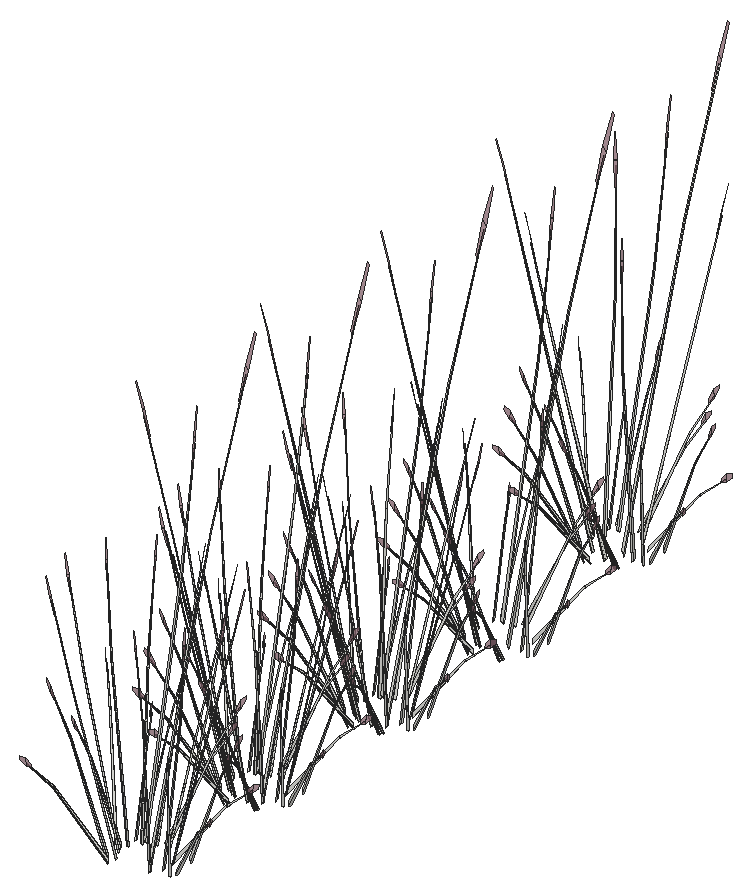
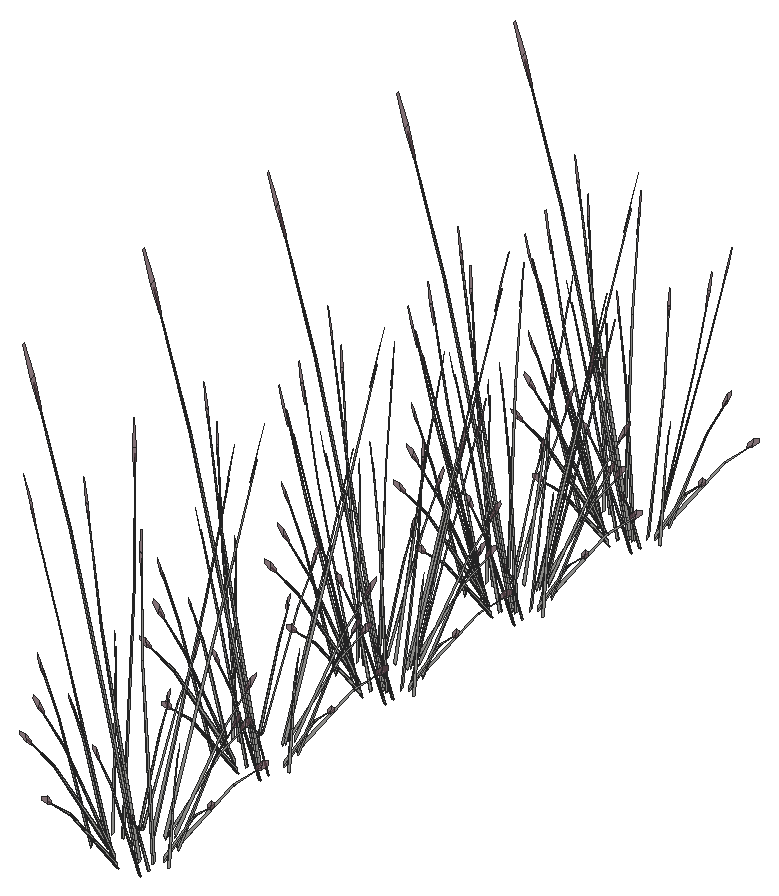
# SketchUp Ruby script. Lengths in inches.
U = 1.inch
M = Sketchup.active_model
def pt(a) = Geom::Point3d.new(a.map { |v| v * U })
def face(e, loops, mat)
  f = e.add_face(loops[0].map { |a| pt(a) })
  loops[1..].each { |l| e.add_face(l.map { |a| pt(a) }).erase! }
  f.material = f.back_material = mat if mat
  f
end
# faces: each face lists its corners as indices into pts; further lists are holes
def faces(e, pts, list, mat = nil) = list.each { |f| face(e, (f[0].is_a?(Array) ? f : [f]).map { |l| l.map { |i| pts[i] } }, mat) }
# xy, xz, yz: faces in a plane at the given z, y or x. An outline is a flat list of corners, or four numbers for a rectangle; further outlines are holes
def ring(l) = l.size == 4 ? [[l[0], l[1]], [l[2], l[1]], [l[2], l[3]], [l[0], l[3]]] : l.each_slice(2).to_a
def flat(e, list, mat, &to3) = list.each { |f| face(e, (f[0].is_a?(Array) ? f : [f]).map { |l| ring(l).map { |u, v| to3.(u, v) } }, mat) }
def xy(e, z, list, mat = nil) = flat(e, list, mat) { |x, y| [x, y, z] }
def xz(e, y, list, mat = nil) = flat(e, list, mat) { |x, z| [x, y, z] }
def yz(e, x, list, mat = nil) = flat(e, list, mat) { |y, z| [x, y, z] }
def lines(e, pts, list) = list.each { |a, b| e.add_line(pt(pts[a]), pt(pts[b])) }
# prism: a flat outline (further loops are holes) pulled along v
def prism(e, loops, v, mat = nil)
  f = face(e, loops, mat); d = Geom::Vector3d.new(v.map { |x| x * U })
  f.pushpull(f.normal.samedirection?(d) ? d.length : -d.length)
end
def box(e, o, s, mat = nil) = prism(e, [[o, [o[0] + s[0], o[1], o[2]], [o[0] + s[0], o[1] + s[1], o[2]], [o[0], o[1] + s[1], o[2]]]], [0, 0, s[2]], mat)
def at(x, y, z, deg = 0) = Geom::Transformation.translation(pt([x, y, z])) * Geom::Transformation.rotation(ORIGIN, Z_AXIS, deg.degrees)
def axes(o, x, y, z) = Geom::Transformation.new([*x, 0, *y, 0, *z, 0, *pt(o).to_a, 1])
def part(name) = M.definitions.add(name)
# library, detail: a bought-in or finely detailed component or shape, given as its bounding box
def library(name, o, s) = part(name).tap { |d| box(d.entities, o, s) }
def detail(e, o, s) = box(e.add_group.entities, o, s)
def put(e, d, t, mat = nil) = e.add_instance(d, t).tap { |i| i.material = mat if mat }
def group(e, t, mat = nil) = e.add_group.tap { |g| g.transformation = t; g.material = mat if mat }.entities
root = M.entities
M.materials.add("LightPink_Translucent").color = [144, 107, 117]
M.materials["LightPink_Translucent"].alpha = 0.75
c1 = part("blade")
p = [[2.15,0.21,22],[0,0.17,0],[0.09,0.45,0],[2.18,0.31,22],[2.29,0.31,22],[0.38,0.45,0],
  [2.48,0.24,33],[2.49,0.24,33],[2.48,0.22,33]]
faces(c1.entities,p,[[0,1,2,3],[4,5,2,3],[6,3,4,7],[8,0,3,6]])
c2 = part("seeds")
p = [[0.3,-0.1,1.38],[-0.01,-0.03,1.59],[-0.01,-0.03,0.03],[0.14,-0.07,-0.07],[0.29,-0.03,3],[0.15,0.01,3.11]]
faces(c2.entities,p,[[0,1,2,3],[1,0,4,5]],"LightPink_Translucent")
c3 = part("blade with seeds")
put(c3.entities,c1,at(0,0,0))
put(c3.entities,c2,axes([2.4,0.25,30.99],[1.5799,-0.05474,1.17369],[-0.12525,1.92788,0.29478],[-0.07173,-0.02425,1.56792]))
put(root,c3,axes([337.34,75.88,268.4],[0.42027,0.02533,0.05988],[-0.01152,0.38243,0.47138],[0.04398,-0.14649,0.71878]))
put(root,c3,axes([333.7,75.16,268.39],[-0.11004,-0.00384,1.62908],[-0.35032,0.38367,-0.25764],[-0.18692,-0.07839,0.13065]))
put(root,c3,axes([339.02,76.93,268.38],[-0.0668,-0.00413,1.65179],[-0.27738,-0.44233,-0.15608],[0.11139,-0.14544,0.29231]))
put(root,c3,axes([333.81,76.02,268.4],[0.02575,-0.41332,0.05988],[0.38885,0.01133,0.47138],[-0.14895,-0.04325,0.71878]))
put(root,c3,axes([338.03,76.95,268.4],[0.35109,0.22859,0.05988],[-0.2044,0.32553,0.47138],[0.11256,-0.10524,0.71878]))
put(root,c3,axes([339.28,77.46,268.39],[0.07097,-0.08279,1.62908],[-0.09083,-0.50786,-0.25764],[0.17806,-0.09629,0.13065]))
put(root,c3,axes([333.28,75.48,268.38],[0.03791,0.05424,1.65179],[-0.18278,0.48761,-0.15608],[-0.18511,0.00353,0.29231]))
put(root,c3,axes([333.21,77.15,268.4],[-0.18783,-0.37061,0.05988],[0.34252,-0.1814,0.47138],[-0.15099,0.03579,0.71878]))
put(root,c3,axes([338.09,78.22,268.4],[0.18783,0.37061,0.05988],[-0.34252,0.1814,0.47138],[0.15099,-0.03579,0.71878]))
put(root,c3,axes([338.9,79.7,268.38],[-0.04624,-0.04758,1.65179],[0.10116,-0.51007,-0.15608],[0.18215,-0.03259,0.29231]))
put(root,c3,axes([332.88,77.625,268.39],[-0.08351,0.07057,1.62908],[0.0071,0.51561,-0.25764],[-0.19143,0.06705,0.13065]))
put(root,c3,axes([337.75,78.92,268.39],[0.10971,-0.00919,1.62908],[0.30091,-0.42228,-0.25764],[0.19514,0.05574,0.13065]))
put(root,c3,axes([333.27,78.42,268.4],[-0.35109,-0.22859,0.05988],[0.2044,-0.32553,0.47138],[-0.11256,0.10524,0.71878]))
put(root,c3,axes([331.96,78.15,268.38],[0.06527,0.01458,1.65179],[0.20191,0.48025,-0.15608],[-0.1336,0.12605,0.29231]))
put(root,c3,axes([337.49,79.35,268.4],[-0.02575,0.41332,0.05988],[-0.38885,-0.01133,0.47138],[0.14895,0.04325,0.71878]))
put(root,c3,axes([336.625,77.11,268.17],[-0.44191,-0.28242,1.28769],[0.46662,-0.43971,0.5556],[0.14258,0.26499,1.24467]))
put(root,c3,axes([335.88,80.24,268.38],[0.00151,-0.06581,1.65179],[0.43826,-0.29033,-0.15608],[0.15223,0.10363,0.29231]))
put(root,c3,axes([333.96,79.49,268.4],[-0.42027,-0.02533,0.05988],[0.01152,-0.38243,0.47138],[-0.04398,0.14649,0.71878]))
put(root,c3,axes([336.39,80.03,268.4],[-0.23243,0.34529,0.05988],[-0.331,-0.20103,0.47138],[0.10701,0.1107,0.71878]))
put(root,c3,axes([335.1,80.08,268.4],[-0.37684,0.18473,0.05988],[-0.18445,-0.33686,0.47138],[0.03639,0.14849,0.71878]))
put(root,c3,axes([332.9,79.55,268.39],[-0.01271,0.10756,1.62908],[0.36076,0.37419,-0.25764],[-0.09444,0.17695,0.13065]))
put(root,c3,axes([334.05,79.31,269.03],[0.56206,0.02693,-0.12569],[-0.01536,0.50991,-0.69765],[-0.03904,0.19638,1.06006]))
put(root,c3,axes([332.86,80.65,268.38],[0.05802,-0.03282,1.65179],[0.47954,0.21828,-0.15608],[-0.01127,0.18175,0.29231]))
put(root,c3,axes([334.97,80.88,268.39],[0.06483,0.08753,1.62908],[0.52315,0.03439,-0.25764],[0.05261,0.19303,0.13065]))
put(root,c3,axes([335.41,89.2,268.39],[-0.07822,-0.07621,1.62908],[-0.52201,0.04832,-0.25764],[-0.08331,-0.18228,0.13065]))
put(root,c3,axes([337.76,90.14,268.39],[-0.00494,-0.10818,1.62908],[-0.41695,-0.31265,-0.25764],[0.06446,-0.18952,0.13065]))
put(root,c3,axes([337.65,89.75,268.38],[-0.05194,0.04152,1.65179],[-0.50886,-0.14007,-0.15608],[-0.01842,-0.18118,0.29231]))
put(root,c3,axes([334.88,88.95,268.38],[-0.00954,0.06515,1.65179],[-0.47055,0.23645,-0.15608],[-0.13847,-0.12087,0.29231]))
put(root,c3,axes([336.2,90.18,268.4],[0.37684,-0.18473,0.05988],[0.18445,0.33686,0.47138],[-0.03639,-0.14849,0.71878]))
put(root,c3,axes([334.91,90.23,268.4],[0.23243,-0.34529,0.05988],[0.331,0.20103,0.47138],[-0.10701,-0.1107,0.71878]))
put(root,c3,axes([335.01,90.19,269.06],[-0.34131,0.52108,-0.12682],[-0.49429,-0.3002,-0.70393],[-0.17182,-0.14722,1.06961]))
put(root,c3,axes([337.34,90.77,268.4],[0.42027,0.02533,0.05988],[-0.01152,0.38243,0.47138],[0.04398,-0.14649,0.71878]))
put(root,c3,axes([333.7,90.04,268.39],[-0.11004,-0.00384,1.62908],[-0.35032,0.38367,-0.25764],[-0.18692,-0.07839,0.13065]))
put(root,c3,axes([339.02,91.82,268.38],[-0.0668,-0.00413,1.65179],[-0.27738,-0.44233,-0.15608],[0.11139,-0.14544,0.29231]))
put(root,c3,axes([333.81,90.91,268.4],[0.02575,-0.41332,0.05988],[0.38885,0.01133,0.47138],[-0.14895,-0.04325,0.71878]))
put(root,c3,axes([338.03,91.84,268.4],[0.35109,0.22859,0.05988],[-0.2044,0.32553,0.47138],[0.11256,-0.10524,0.71878]))
put(root,c3,axes([339.28,92.35,268.39],[0.07097,-0.08279,1.62908],[-0.09083,-0.50786,-0.25764],[0.17806,-0.09629,0.13065]))
put(root,c3,axes([333.28,90.37,268.38],[0.03791,0.05424,1.65179],[-0.18278,0.48761,-0.15608],[-0.18511,0.00353,0.29231]))
put(root,c3,axes([333.21,92.03,268.4],[-0.18783,-0.37061,0.05988],[0.34252,-0.1814,0.47138],[-0.15099,0.03579,0.71878]))
put(root,c3,axes([338.09,93.11,268.4],[0.18783,0.37061,0.05988],[-0.34252,0.1814,0.47138],[0.15099,-0.03579,0.71878]))
put(root,c3,axes([338.9,94.58,268.38],[-0.04624,-0.04758,1.65179],[0.10116,-0.51007,-0.15608],[0.18215,-0.03259,0.29231]))
put(root,c3,axes([332.88,92.51,268.39],[-0.08351,0.07057,1.62908],[0.0071,0.51561,-0.25764],[-0.19143,0.06705,0.13065]))
put(root,c3,axes([337.75,93.8125,268.39],[0.10971,-0.00919,1.62908],[0.30091,-0.42228,-0.25764],[0.19514,0.05574,0.13065]))
put(root,c3,axes([333.27,93.3,268.4],[-0.35109,-0.22859,0.05988],[0.2044,-0.32553,0.47138],[-0.11256,0.10524,0.71878]))
put(root,c3,axes([331.96,93.03,268.38],[0.06527,0.01458,1.65179],[0.20191,0.48025,-0.15608],[-0.1336,0.12605,0.29231]))
put(root,c3,axes([337.49,94.24,268.4],[-0.02575,0.41332,0.05988],[-0.38885,-0.01133,0.47138],[0.14895,0.04325,0.71878]))
put(root,c3,axes([336.625,92,268.17],[-0.44191,-0.28242,1.28769],[0.46662,-0.43971,0.5556],[0.14258,0.26499,1.24467]))
put(root,c3,axes([335.88,95.13,268.38],[0.00151,-0.06581,1.65179],[0.43826,-0.29033,-0.15608],[0.15223,0.10363,0.29231]))
put(root,c3,axes([333.96,94.375,268.4],[-0.42027,-0.02533,0.05988],[0.01152,-0.38243,0.47138],[-0.04398,0.14649,0.71878]))
put(root,c3,axes([336.39,94.91,268.4],[-0.23243,0.34529,0.05988],[-0.331,-0.20103,0.47138],[0.10701,0.1107,0.71878]))
put(root,c3,axes([335.1,94.97,268.4],[-0.37684,0.18473,0.05988],[-0.18445,-0.33686,0.47138],[0.03639,0.14849,0.71878]))
put(root,c3,axes([332.9,94.4375,268.39],[-0.01271,0.10756,1.62908],[0.36076,0.37419,-0.25764],[-0.09444,0.17695,0.13065]))
put(root,c3,axes([334.05,94.2,269.03],[0.56206,0.02693,-0.12569],[-0.01536,0.50991,-0.69765],[-0.03904,0.19638,1.06006]))
put(root,c3,axes([332.86,95.54,268.38],[0.05802,-0.03282,1.65179],[0.47954,0.21828,-0.15608],[-0.01127,0.18175,0.29231]))
put(root,c3,axes([334.97,95.77,268.39],[0.06483,0.08753,1.62908],[0.52315,0.03439,-0.25764],[0.05261,0.19303,0.13065]))
put(root,c3,axes([335.41,105.62,268.39],[-0.07822,-0.07621,1.62908],[-0.52201,0.04832,-0.25764],[-0.08331,-0.18228,0.13065]))
put(root,c3,axes([337.76,106.56,268.39],[-0.00494,-0.10818,1.62908],[-0.41695,-0.31265,-0.25764],[0.06446,-0.18952,0.13065]))
put(root,c3,axes([337.65,106.17,268.38],[-0.05194,0.04152,1.65179],[-0.50886,-0.14007,-0.15608],[-0.01842,-0.18118,0.29231]))
put(root,c3,axes([334.88,105.37,268.38],[-0.00954,0.06515,1.65179],[-0.47055,0.23645,-0.15608],[-0.13847,-0.12087,0.29231]))
put(root,c3,axes([336.2,106.59,268.4],[0.37684,-0.18473,0.05988],[0.18445,0.33686,0.47138],[-0.03639,-0.14849,0.71878]))
put(root,c3,axes([334.91,106.65,268.4],[0.23243,-0.34529,0.05988],[0.331,0.20103,0.47138],[-0.10701,-0.1107,0.71878]))
put(root,c3,axes([335.01,106.61,269.06],[-0.34131,0.52108,-0.12682],[-0.49429,-0.3002,-0.70393],[-0.17182,-0.14722,1.06961]))
put(root,c3,axes([337.34,107.18,268.4],[0.42027,0.02533,0.05988],[-0.01152,0.38243,0.47138],[0.04398,-0.14649,0.71878]))
put(root,c3,axes([333.7,106.46,268.39],[-0.11004,-0.00384,1.62908],[-0.35032,0.38367,-0.25764],[-0.18692,-0.07839,0.13065]))
put(root,c3,axes([339.02,108.24,268.38],[-0.0668,-0.00413,1.65179],[-0.27738,-0.44233,-0.15608],[0.11139,-0.14544,0.29231]))
put(root,c3,axes([333.81,107.33,268.4],[0.02575,-0.41332,0.05988],[0.38885,0.01133,0.47138],[-0.14895,-0.04325,0.71878]))
put(root,c3,axes([338.03,108.26,268.4],[0.35109,0.22859,0.05988],[-0.2044,0.32553,0.47138],[0.11256,-0.10524,0.71878]))
put(root,c3,axes([339.28,108.77,268.39],[0.07097,-0.08279,1.62908],[-0.09083,-0.50786,-0.25764],[0.17806,-0.09629,0.13065]))
put(root,c3,axes([333.28,106.79,268.38],[0.03791,0.05424,1.65179],[-0.18278,0.48761,-0.15608],[-0.18511,0.00353,0.29231]))
put(root,c3,axes([333.21,108.45,268.4],[-0.18783,-0.37061,0.05988],[0.34252,-0.1814,0.47138],[-0.15099,0.03579,0.71878]))
put(root,c3,axes([338.09,109.53,268.4],[0.18783,0.37061,0.05988],[-0.34252,0.1814,0.47138],[0.15099,-0.03579,0.71878]))
put(root,c3,axes([338.9,111,268.38],[-0.04624,-0.04758,1.65179],[0.10116,-0.51007,-0.15608],[0.18215,-0.03259,0.29231]))
put(root,c3,axes([332.88,108.93,268.39],[-0.08351,0.07057,1.62908],[0.0071,0.51561,-0.25764],[-0.19143,0.06705,0.13065]))
put(root,c3,axes([337.75,110.23,268.39],[0.10971,-0.00919,1.62908],[0.30091,-0.42228,-0.25764],[0.19514,0.05574,0.13065]))
put(root,c3,axes([333.27,109.72,268.4],[-0.35109,-0.22859,0.05988],[0.2044,-0.32553,0.47138],[-0.11256,0.10524,0.71878]))
put(root,c3,axes([331.96,109.45,268.38],[0.06527,0.01458,1.65179],[0.20191,0.48025,-0.15608],[-0.1336,0.12605,0.29231]))
put(root,c3,axes([337.49,110.65,268.4],[-0.02575,0.41332,0.05988],[-0.38885,-0.01133,0.47138],[0.14895,0.04325,0.71878]))
put(root,c3,axes([336.625,108.42,268.17],[-0.44191,-0.28242,1.28769],[0.46662,-0.43971,0.5556],[0.14258,0.26499,1.24467]))
put(root,c3,axes([335.88,111.55,268.38],[0.00151,-0.06581,1.65179],[0.43826,-0.29033,-0.15608],[0.15223,0.10363,0.29231]))
put(root,c3,axes([333.96,110.79,268.4],[-0.42027,-0.02533,0.05988],[0.01152,-0.38243,0.47138],[-0.04398,0.14649,0.71878]))
put(root,c3,axes([336.39,111.33,268.4],[-0.23243,0.34529,0.05988],[-0.331,-0.20103,0.47138],[0.10701,0.1107,0.71878]))
put(root,c3,axes([335.1,111.38,268.4],[-0.37684,0.18473,0.05988],[-0.18445,-0.33686,0.47138],[0.03639,0.14849,0.71878]))
put(root,c3,axes([332.9,110.86,268.39],[-0.01271,0.10756,1.62908],[0.36076,0.37419,-0.25764],[-0.09444,0.17695,0.13065]))
put(root,c3,axes([334.05,110.61,269.03],[0.56206,0.02693,-0.12569],[-0.01536,0.50991,-0.69765],[-0.03904,0.19638,1.06006]))
put(root,c3,axes([332.86,111.96,268.38],[0.05802,-0.03282,1.65179],[0.47954,0.21828,-0.15608],[-0.01127,0.18175,0.29231]))
put(root,c3,axes([334.97,112.1875,268.39],[0.06483,0.08753,1.62908],[0.52315,0.03439,-0.25764],[0.05261,0.19303,0.13065]))
put(root,c3,axes([335.41,121.46,268.39],[-0.07822,-0.07621,1.62908],[-0.52201,0.04832,-0.25764],[-0.08331,-0.18228,0.13065]))
put(root,c3,axes([337.76,122.39,268.39],[-0.00494,-0.10818,1.62908],[-0.41695,-0.31265,-0.25764],[0.06446,-0.18952,0.13065]))
put(root,c3,axes([337.65,122.01,268.38],[-0.05194,0.04152,1.65179],[-0.50886,-0.14007,-0.15608],[-0.01842,-0.18118,0.29231]))
put(root,c3,axes([334.88,121.21,268.38],[-0.00954,0.06515,1.65179],[-0.47055,0.23645,-0.15608],[-0.13847,-0.12087,0.29231]))
put(root,c3,axes([334.91,122.49,268.4],[0.23243,-0.34529,0.05988],[0.331,0.20103,0.47138],[-0.10701,-0.1107,0.71878]))
put(root,c3,axes([335.01,122.45,269.06],[-0.34131,0.52108,-0.12682],[-0.49429,-0.3002,-0.70393],[-0.17182,-0.14722,1.06961]))
put(root,c3,axes([333.7,122.3,268.39],[-0.11004,-0.00384,1.62908],[-0.35032,0.38367,-0.25764],[-0.18692,-0.07839,0.13065]))
put(root,c3,axes([339.02,124.08,268.38],[-0.0668,-0.00413,1.65179],[-0.27738,-0.44233,-0.15608],[0.11139,-0.14544,0.29231]))
put(root,c3,axes([338.03,124.1,268.4],[0.35109,0.22859,0.05988],[-0.2044,0.32553,0.47138],[0.11256,-0.10524,0.71878]))
put(root,c3,axes([339.28,124.61,268.39],[0.07097,-0.08279,1.62908],[-0.09083,-0.50786,-0.25764],[0.17806,-0.09629,0.13065]))
put(root,c3,axes([333.28,122.625,268.38],[0.03791,0.05424,1.65179],[-0.18278,0.48761,-0.15608],[-0.18511,0.00353,0.29231]))
put(root,c3,axes([338.9,126.84,268.38],[-0.04624,-0.04758,1.65179],[0.10116,-0.51007,-0.15608],[0.18215,-0.03259,0.29231]))
put(root,c3,axes([332.88,124.77,268.39],[-0.08351,0.07057,1.62908],[0.0071,0.51561,-0.25764],[-0.19143,0.06705,0.13065]))
put(root,c3,axes([337.75,126.07,268.39],[0.10971,-0.00919,1.62908],[0.30091,-0.42228,-0.25764],[0.19514,0.05574,0.13065]))
put(root,c3,axes([331.96,125.29,268.38],[0.06527,0.01458,1.65179],[0.20191,0.48025,-0.15608],[-0.1336,0.12605,0.29231]))
put(root,c3,axes([336.625,124.26,268.17],[-0.44191,-0.28242,1.28769],[0.46662,-0.43971,0.5556],[0.14258,0.26499,1.24467]))
put(root,c3,axes([335.88,127.39,268.38],[0.00151,-0.06581,1.65179],[0.43826,-0.29033,-0.15608],[0.15223,0.10363,0.29231]))
put(root,c3,axes([335.1,127.22,268.4],[-0.37684,0.18473,0.05988],[-0.18445,-0.33686,0.47138],[0.03639,0.14849,0.71878]))
put(root,c3,axes([332.9,126.7,268.39],[-0.01271,0.10756,1.62908],[0.36076,0.37419,-0.25764],[-0.09444,0.17695,0.13065]))
put(root,c3,axes([334.05,126.45,269.03],[0.56206,0.02693,-0.12569],[-0.01536,0.50991,-0.69765],[-0.03904,0.19638,1.06006]))
put(root,c3,axes([332.86,127.8,268.38],[0.05802,-0.03282,1.65179],[0.47954,0.21828,-0.15608],[-0.01127,0.18175,0.29231]))
put(root,c3,axes([334.97,128.03,268.39],[0.06483,0.08753,1.62908],[0.52315,0.03439,-0.25764],[0.05261,0.19303,0.13065]))
put(root,c3,axes([333.2,139.47,268.39],[-0.07822,-0.07621,1.62908],[-0.52201,0.04832,-0.25764],[-0.08331,-0.18228,0.13065]))
put(root,c3,axes([335.54,140.4,268.39],[-0.00494,-0.10818,1.62908],[-0.41695,-0.31265,-0.25764],[0.06446,-0.18952,0.13065]))
put(root,c3,axes([335.43,140.02,268.38],[-0.05194,0.04152,1.65179],[-0.50886,-0.14007,-0.15608],[-0.01842,-0.18118,0.29231]))
put(root,c3,axes([332.66,139.22,268.38],[-0.00954,0.06515,1.65179],[-0.47055,0.23645,-0.15608],[-0.13847,-0.12087,0.29231]))
put(root,c3,axes([333.99,140.65,268.6875],[-0.50045,0.25306,-0.11324],[-0.24593,-0.44915,-0.62851],[-0.06603,-0.18927,0.95501]))
put(root,c3,axes([332.8,140.46,269.06],[-0.34131,0.52108,-0.12682],[-0.49429,-0.3002,-0.70393],[-0.17182,-0.14722,1.06961]))
put(root,c3,axes([331.49,140.31,268.39],[-0.11004,-0.00384,1.62908],[-0.35032,0.38367,-0.25764],[-0.18692,-0.07839,0.13065]))
put(root,c3,axes([335.64,142.22,268.6875],[-0.47307,-0.29971,-0.11324],[0.27254,-0.43404,-0.62851],[0.13365,-0.15087,0.95501]))
put(root,c3,axes([336.81,142.09,268.38],[-0.0668,-0.00413,1.65179],[-0.27738,-0.44233,-0.15608],[0.11139,-0.14544,0.29231]))
put(root,c3,axes([337.0625,142.62,268.39],[0.07097,-0.08279,1.62908],[-0.09083,-0.50786,-0.25764],[0.17806,-0.09629,0.13065]))
put(root,c3,axes([331.0625,140.63,268.38],[0.03791,0.05424,1.65179],[-0.18278,0.48761,-0.15608],[-0.18511,0.00353,0.29231]))
put(root,c3,axes([336.6875,144.85,268.38],[-0.04624,-0.04758,1.65179],[0.10116,-0.51007,-0.15608],[0.18215,-0.03259,0.29231]))
put(root,c3,axes([330.67,142.78,268.39],[-0.08351,0.07057,1.62908],[0.0071,0.51561,-0.25764],[-0.19143,0.06705,0.13065]))
put(root,c3,axes([335.54,144.08,268.39],[0.10971,-0.00919,1.62908],[0.30091,-0.42228,-0.25764],[0.19514,0.05574,0.13065]))
put(root,c3,axes([329.74,143.3,268.38],[0.06527,0.01458,1.65179],[0.20191,0.48025,-0.15608],[-0.1336,0.12605,0.29231]))
put(root,c3,axes([334.41,142.27,268.17],[-0.44191,-0.28242,1.28769],[0.46662,-0.43971,0.5556],[0.14258,0.26499,1.24467]))
put(root,c3,axes([331.22,143.46,268.6875],[0.47307,0.29971,-0.11324],[-0.27254,0.43404,-0.62851],[-0.13365,0.15087,0.95501]))
put(root,c3,axes([334.06,145.01,268.6875],[0.30474,-0.46525,-0.11324],[0.44133,0.26804,-0.62851],[0.15341,0.13145,0.95501]))
put(root,c3,axes([333.67,145.4,268.38],[0.00151,-0.06581,1.65179],[0.43826,-0.29033,-0.15608],[0.15223,0.10363,0.29231]))
put(root,c3,axes([330.68,144.71,268.39],[-0.01271,0.10756,1.62908],[0.36076,0.37419,-0.25764],[-0.09444,0.17695,0.13065]))
put(root,c3,axes([331.84,144.46,269.03],[0.56206,0.02693,-0.12569],[-0.01536,0.50991,-0.69765],[-0.03904,0.19638,1.06006]))
put(root,c3,axes([330.64,145.81,268.38],[0.05802,-0.03282,1.65179],[0.47954,0.21828,-0.15608],[-0.01127,0.18175,0.29231]))
put(root,c3,axes([332.76,146.04,268.39],[0.06483,0.08753,1.62908],[0.52315,0.03439,-0.25764],[0.05261,0.19303,0.13065]))
